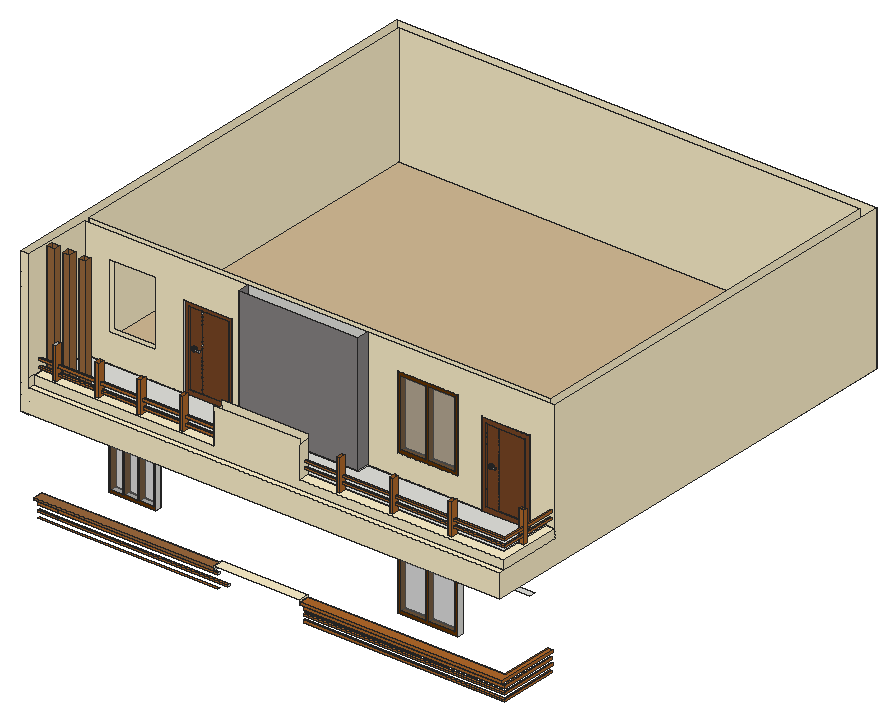
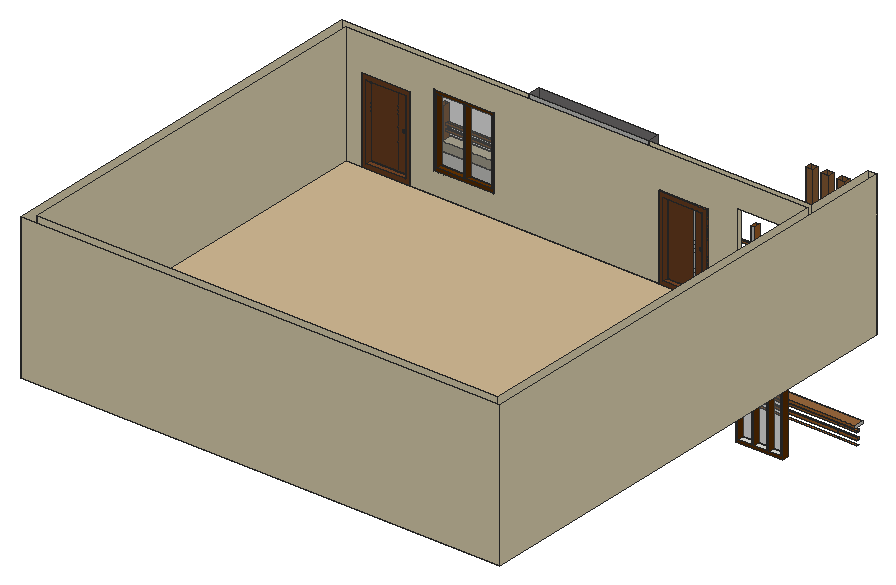
# SketchUp Ruby script. Lengths in inches.
U = 1.inch
M = Sketchup.active_model
def pt(a) = Geom::Point3d.new(a.map { |v| v * U })
def face(e, loops, mat)
  f = e.add_face(loops[0].map { |a| pt(a) })
  loops[1..].each { |l| e.add_face(l.map { |a| pt(a) }).erase! }
  f.material = f.back_material = mat if mat
  f
end
# faces: each face lists its corners as indices into pts; further lists are holes
def faces(e, pts, list, mat = nil) = list.each { |f| face(e, (f[0].is_a?(Array) ? f : [f]).map { |l| l.map { |i| pts[i] } }, mat) }
# xy, xz, yz: faces in a plane at the given z, y or x. An outline is a flat list of corners, or four numbers for a rectangle; further outlines are holes
def ring(l) = l.size == 4 ? [[l[0], l[1]], [l[2], l[1]], [l[2], l[3]], [l[0], l[3]]] : l.each_slice(2).to_a
def flat(e, list, mat, &to3) = list.each { |f| face(e, (f[0].is_a?(Array) ? f : [f]).map { |l| ring(l).map { |u, v| to3.(u, v) } }, mat) }
def xy(e, z, list, mat = nil) = flat(e, list, mat) { |x, y| [x, y, z] }
def xz(e, y, list, mat = nil) = flat(e, list, mat) { |x, z| [x, y, z] }
def yz(e, x, list, mat = nil) = flat(e, list, mat) { |y, z| [x, y, z] }
def lines(e, pts, list) = list.each { |a, b| e.add_line(pt(pts[a]), pt(pts[b])) }
# prism: a flat outline (further loops are holes) pulled along v
def prism(e, loops, v, mat = nil)
  f = face(e, loops, mat); d = Geom::Vector3d.new(v.map { |x| x * U })
  f.pushpull(f.normal.samedirection?(d) ? d.length : -d.length)
end
def box(e, o, s, mat = nil) = prism(e, [[o, [o[0] + s[0], o[1], o[2]], [o[0] + s[0], o[1] + s[1], o[2]], [o[0], o[1] + s[1], o[2]]]], [0, 0, s[2]], mat)
def at(x, y, z, deg = 0) = Geom::Transformation.translation(pt([x, y, z])) * Geom::Transformation.rotation(ORIGIN, Z_AXIS, deg.degrees)
def axes(o, x, y, z) = Geom::Transformation.new([*x, 0, *y, 0, *z, 0, *pt(o).to_a, 1])
def part(name) = M.definitions.add(name)
# library, detail: a bought-in or finely detailed component or shape, given as its bounding box
def library(name, o, s) = part(name).tap { |d| box(d.entities, o, s) }
def detail(e, o, s) = box(e.add_group.entities, o, s)
def put(e, d, t, mat = nil) = e.add_instance(d, t).tap { |i| i.material = mat if mat }
def group(e, t, mat = nil) = e.add_group.tap { |g| g.transformation = t; g.material = mat if mat }.entities
root = M.entities
M.materials.add("[Aluminum]").color = [179, 179, 179]
M.materials.add("[Brick Tumbled]").color = [135, 132, 132]
M.materials.add("[Color C08]").color = [102, 51, 0]
M.materials.add("[Color D01]").color = [255, 242, 204]
M.materials.add("[Formica Beige]").color = [211, 187, 149]
M.materials.add("[Translucent Glass Gray]").color = [128, 128, 128]
M.materials["[Translucent Glass Gray]"].alpha = 0.5
M.materials.add("[Wood Bamboo]").color = [177, 105, 43]
M.materials.add("[Wood Floor]").color = [155, 105, 61]
M.materials.add("[Wood Veneer 01]").color = [120, 70, 37]
c1 = part("Group\#4")
xy(c1.entities,0,[[0,0,52.875,9]],"[Color C08]")
xy(c1.entities,2.31,[[2.31,0,24.96,9],[26.98,0,50.56,9]],"[Color C08]")
xy(c1.entities,50.56,[[2.31,0,24.96,9],[26.98,0,50.56,9]],"[Color C08]")
xy(c1.entities,52.875,[[0,0,52.875,9]],"[Color C08]")
xz(c1.entities,0,[[[0,0,52.875,52.875],[26.98,2.31,50.56,50.56],[2.31,2.31,24.96,50.56]]],"[Color C08]")
xz(c1.entities,0,[[2.31,2.31,24.96,50.56],[26.98,2.31,50.56,50.56]],"[Translucent Glass Gray]")
xz(c1.entities,9,[[[0,0,52.875,52.875],[26.98,2.31,50.56,50.56],[2.31,2.31,24.96,50.56]]],"[Color C08]")
yz(c1.entities,0,[[0,0,9,52.875]],"[Color C08]")
yz(c1.entities,2.31,[[0,2.31,9,50.56]],"[Color C08]")
yz(c1.entities,24.96,[[0,2.31,9,50.56]],"[Color C08]")
yz(c1.entities,26.98,[[0,2.31,9,50.56]],"[Color C08]")
yz(c1.entities,50.56,[[0,2.31,9,50.56]],"[Color C08]")
yz(c1.entities,52.875,[[0,0,9,52.875]],"[Color C08]")
xy(root,309.67,[[322.9,204.4,382.78,210.4]])
xy(root,310.18,[[274.98,145.89,274.98,148.02,475.1875,148.02,475.1875,204.4,477.01,204.4,477.01,145.89]],"[Wood Bamboo]")
xy(root,310.55,[[9,146.02,28.82,148.14],[28.82,146.02,189.63,148.14]],"[Wood Bamboo]")
xy(root,312.3,[[274.98,145.89,477.01,145.89,477.01,204.4,475.1875,204.4,475.1875,148.02,274.98,148.02]],"[Wood Bamboo]")
xy(root,315.61,[[9,146.02,28.82,148.14]])
xy(root,315.61,[[28.82,146.02,199.2,148.14]],"[Wood Bamboo]")
xy(root,316.36,[[274.98,145.89,274.98,148.02,475.1875,148.02,475.1875,205.64,477.01,205.64,477.01,145.89]],"[Wood Bamboo]")
xy(root,316.68,[[33.82,204.4,80.13,210.4]])
xy(root,317.73,[[9,146.02,28.82,148.14],[28.82,146.02,199.2,148.14]],"[Wood Bamboo]")
xy(root,318.49,[[274.98,145.89,477.01,145.89,477.01,205.64,475.1875,205.64,475.1875,148.02,274.98,148.02]],"[Wood Bamboo]")
xy(root,321.93,[[274.98,145.89,274.98,148.02,475.1875,148.02,475.1875,204.36,477.01,204.36,477.01,145.89]],"[Wood Bamboo]")
xy(root,322.48,[[9,146.02,28.82,148.14]])
xy(root,322.48,[[28.82,146.02,189.2,148.14]],"[Wood Bamboo]")
xy(root,324.43,[[274.98,145.89,477.01,145.89,477.01,204.36,475.1875,204.36,475.1875,148.02,274.98,148.02]],"[Wood Bamboo]")
xy(root,324.61,[[9,146.02,28.82,148.14],[28.82,146.02,189.2,148.14]],"[Wood Bamboo]")
xy(root,327.9375,[[309.7,143.88,313.07,150.13]])
xy(root,328.12,[[[8.16,141.71,188.91,151.78],[68.13,143.88,71.51,150.13],[110.26,143.88,113.63,150.13]],[[274.98,141.71,274.98,151.78,472.375,151.78,472.375,205.65,477.34,205.65,477.34,141.71],[421.51,143.88,424.88,150.13]]],"[Wood Bamboo]")
xy(root,328.125,[[472.3125,168.86,477.25,172.24]])
xy(root,328.375,[[152.95,143.88,156.32,150.13]])
xy(root,328.5,[[362.95,143.88,366.32,150.13]])
xy(root,328.9375,[[25.45,143.88,28.82,150.13]])
xy(root,330.66,[[274.98,141.71,477.34,141.71,477.34,205.65,472.375,205.65,472.375,151.78,274.98,151.78]],"[Wood Bamboo]")
xy(root,330.66,[[8.16,141.71,188.91,151.78]],"[Wood Floor]")
xy(root,332.875,[[188.91,140.9,274.98,151.78]],"[Color D01]")
xy(root,371.875,[[108.75,204.4,156.75,210.4],[407.0625,204.4,455.0625,210.4]])
xy(root,382.5,[[33.82,204.4,80.13,210.4]])
xy(root,382.8,[[322.9,204.4,382.78,210.4]])
xy(root,407.875,[[0,135.4,480,606.75]])
xy(root,407.875,[[172.75,192.4,292.75,204.4]],"[Brick Tumbled]")
xy(root,407.875,[[[0,135.4,9,135.4,9,204.4,480,204.4,480,606.75,0,606.75],[9,210.4,471,597.75]]],"[Color D01]")
xy(root,407.875,[[11.75,154.17,19.6875,160.61],[27.8125,154.17,35,160.61],[43.5625,154.17,50.1875,160.61]],"[Wood Floor]")
xy(root,420.875,[[9,151.78,9,204.4,108.75,204.4,108.75,210.4,156.75,210.4,156.75,204.4,172.75,204.4,172.75,192.4,292.75,192.4,292.75,204.4,407.0625,204.4,407.0625,210.4,455.0625,210.4,455.0625,204.4,471,204.4,471,151.78]])
xy(root,431.8125,[[9,140.9,9,151.78,471,151.78,471,204.4,480,204.4,480,140.9],[[9,151.78,471,151.78,471,204.4,455.0625,204.4,455.0625,210.4,407.0625,210.4,407.0625,204.4,292.75,204.4,292.75,192.4,172.75,192.4,172.75,204.4,156.75,204.4,156.75,210.4,108.75,210.4,108.75,204.4,9,204.4],[11.75,154.17,19.6875,160.61],[27.8125,154.17,35,160.61],[43.5625,154.17,50.1875,160.61]],[172.75,192.4,292.75,204.4],[156.75,204.4,407.0625,210.4]])
xy(root,431.8125,[[9,135.4,480,140.9]],"[Color D01]")
xy(root,431.8125,[[9,210.4,471,597.75]],"[Formica Beige]")
xy(root,440.8125,[[[9,140.9,188.91,151.78],[25.45,143.88,28.82,150.13],[68.13,143.88,71.51,150.13],[110.26,143.88,113.63,150.13],[152.95,143.88,156.32,150.13]],[[274.98,140.9,480,140.9,480,204.4,471,204.4,471,151.78,274.98,151.78],[309.7,143.88,313.07,150.13],[421.51,143.88,424.88,150.13],[362.95,143.88,366.32,150.13],[472.3125,168.86,477.25,172.24]]],"[Color D01]")
xy(root,445.02,[[9,146.22,28.82,148.34]])
xy(root,445.02,[[28.82,146.22,188.91,148.34]],"[Wood Bamboo]")
xy(root,447.15,[[9,146.22,28.82,148.34],[28.82,146.22,188.91,148.34]],"[Wood Bamboo]")
xy(root,447.99,[[274.98,145.89,274.98,148.02,475.1875,148.02,475.1875,207.71,477.01,207.71,477.01,145.89]],"[Wood Bamboo]")
xy(root,450.11,[[274.98,145.89,477.01,145.89,477.01,207.71,475.1875,207.71,475.1875,148.02,274.98,148.02]],"[Wood Bamboo]")
xy(root,452.36,[[9,146.02,28.82,148.14]])
xy(root,452.36,[[28.82,146.02,189.63,148.14]],"[Wood Bamboo]")
xy(root,453.61,[[322.9,204.4,382.78,210.4]])
xy(root,454.11,[[274.98,145.89,274.98,148.02,475.1875,148.02,475.1875,204.4,477.01,204.4,477.01,145.89]],"[Wood Bamboo]")
xy(root,454.48,[[9,146.02,28.82,148.14],[28.82,146.02,189.63,148.14]],"[Wood Bamboo]")
xz(root,135.4,[[0,407.875,480,407.875,480,431.8125,9,431.8125,9,551.8125,0,551.8125]],"[Color D01]")
xz(root,140.9,[[9,431.8125,480,431.8125,480,440.8125,274.98,440.8125,274.98,476.8125,188.91,476.8125,188.91,440.8125,9,440.8125]],"[Color D01]")
xz(root,141.71,[[274.98,328.12,477.34,330.66]],"[Wood Bamboo]")
xz(root,141.71,[[8.16,328.12,188.91,330.66]],"[Wood Floor]")
xz(root,143.88,[[25.45,440.8125,28.82,472.875],[68.13,440.8125,71.51,472.05],[110.26,440.8125,113.63,472.05],[152.95,440.8125,156.32,472.3125],[309.7,440.8125,313.07,471.875],
  [362.95,440.8125,366.32,472.4375],[421.51,440.8125,424.88,472.05]],"[Wood Bamboo]")
xz(root,145.89,[[274.98,310.18,477.01,312.3],[274.98,316.36,477.01,318.49],[274.98,321.93,477.01,324.43],[274.98,447.99,477.01,450.11],[274.98,454.11,477.01,456.24]],"[Wood Bamboo]")
xz(root,146.02,[[9,315.61,28.82,317.73],[28.82,315.61,199.2,317.73],[9,322.48,28.82,324.61],[28.82,322.48,189.2,324.61],[9,452.36,28.82,454.48],
  [28.82,452.36,189.63,454.48]],"[Wood Bamboo]")
xz(root,146.22,[[9,445.02,28.82,447.15],[28.82,445.02,188.91,447.15]],"[Wood Bamboo]")
xz(root,148.02,[[274.98,310.18,475.1875,312.3],[274.98,316.36,475.1875,318.49],[274.98,321.93,475.1875,324.43],[274.98,447.99,475.1875,450.11],[274.98,454.11,475.1875,456.24]],"[Wood Bamboo]")
xz(root,148.14,[[9,315.61,28.82,317.73],[28.82,315.61,199.2,317.73],[9,322.48,28.82,324.61],[28.82,322.48,189.2,324.61],[9,452.36,28.82,454.48],
  [28.82,452.36,189.63,454.48]],"[Wood Bamboo]")
xz(root,148.34,[[9,445.02,28.82,447.15],[28.82,445.02,188.91,447.15]],"[Wood Bamboo]")
xz(root,150.13,[[110.26,440.8125,113.63,472.05],[152.95,440.8125,156.32,472.3125]])
xz(root,150.13,[[25.45,440.8125,28.82,472.875],[68.13,440.8125,71.51,472.05],[309.7,440.8125,313.07,471.875],[362.95,440.8125,366.32,472.4375],[421.51,440.8125,424.88,472.05]],"[Wood Bamboo]")
xz(root,151.78,[[9,420.875,471,431.8125]])
xz(root,151.78,[[9,431.8125,9,440.8125,188.91,440.8125,188.91,476.8125,274.98,476.8125,274.98,440.8125,471,440.8125,471,431.8125]],"[Color D01]")
xz(root,151.78,[[8.16,328.12,188.91,330.66],[274.98,328.12,472.375,330.66]],"[Wood Bamboo]")
xz(root,154.17,[[11.75,431.8125,19.6875,551.8125],[27.8125,431.8125,35,551.8125],[43.5625,431.8125,50.1875,551.8125]],"[Wood Floor]")
xz(root,160.61,[[11.75,431.8125,19.6875,551.8125],[27.8125,431.8125,35,551.8125],[43.5625,431.8125,50.1875,551.8125]],"[Wood Floor]")
xz(root,168.86,[[472.3125,440.8125,477.25,472.0625]],"[Wood Bamboo]")
xz(root,172.24,[[472.3125,440.8125,477.25,472.0625]],"[Wood Bamboo]")
xz(root,192.4,[[172.75,420.875,292.75,431.8125]])
xz(root,192.4,[[172.75,431.8125,292.75,551.8125]],"[Brick Tumbled]")
xz(root,204.36,[[475.1875,321.93,477.01,324.43]])
xz(root,204.4,[[9,420.875,108.75,431.8125],[156.75,420.875,172.75,431.8125],[292.75,420.875,407.0625,431.8125],[455.0625,420.875,471,431.8125],[172.75,431.8125,292.75,551.8125],
  [471,431.8125,480,440.8125]])
xz(root,204.4,[[[9,431.8125,108.75,431.8125,108.75,515.8125,156.75,515.8125,156.75,431.8125,172.75,431.8125,172.75,551.8125,9,551.8125],[33.82,460.62,80.13,526.43]],[[292.75,431.8125,407.0625,431.8125,407.0625,515.8125,455.0625,515.8125,455.0625,431.8125,471,431.8125,471,440.8125,480,440.8125,480,551.8125,292.75,551.8125],[322.9,453.61,382.78,526.73],[475.1875,454.11,477.01,456.24]]],"[Color D01]")
xz(root,205.64,[[475.1875,316.36,477.01,318.49]])
xz(root,205.65,[[472.375,328.12,477.34,330.66]])
xz(root,207.71,[[475.1875,447.99,477.01,450.11]])
xz(root,210.4,[[108.75,420.875,156.75,431.8125],[407.0625,420.875,455.0625,431.8125]])
xz(root,210.4,[[[9,431.8125,9,551.8125,471,551.8125,471,431.8125,455.0625,431.8125,455.0625,515.8125,407.0625,515.8125,407.0625,431.8125,156.75,431.8125,156.75,515.8125,108.75,515.8125,108.75,431.8125],[322.9,453.61,382.78,526.73],[33.82,460.62,80.13,526.43]]],"[Color D01]")
xz(root,597.75,[[9,431.8125,471,551.8125]],"[Color D01]")
xz(root,606.75,[[0,407.875,480,551.8125]],"[Color D01]")
yz(root,0,[[135.4,407.875,606.75,551.8125]],"[Color D01]")
yz(root,8.16,[[141.71,328.12,151.78,330.66]])
yz(root,9,[[151.78,420.875,204.4,431.8125],[140.9,431.8125,151.78,440.8125]])
yz(root,9,[[135.4,431.8125,140.9,440.8125],[[151.78,431.8125,204.4,431.8125,204.4,551.8125,135.4,551.8125,135.4,440.8125,151.78,440.8125],[146.02,466.42,148.14,468.55],[146.02,459.55,148.14,461.67],[146.02,452.36,148.14,454.48],[146.22,445.02,148.34,447.15]],[210.4,431.8125,597.75,551.8125]],"[Color D01]")
yz(root,11.75,[[154.17,431.8125,160.61,551.8125]],"[Wood Floor]")
yz(root,19.6875,[[154.17,431.8125,160.61,551.8125]],"[Wood Floor]")
yz(root,25.45,[[143.88,440.8125,150.13,472.875]])
yz(root,27.8125,[[154.17,431.8125,160.61,551.8125]],"[Wood Floor]")
yz(root,28.82,[[146.02,315.61,148.14,317.73],[146.02,322.48,148.14,324.61],[146.22,445.02,148.34,447.15],[146.02,452.36,148.14,454.48]])
yz(root,28.82,[[[143.88,440.8125,150.13,472.875],[146.02,466.42,148.14,468.55],[146.02,459.55,148.14,461.67],[146.02,452.36,148.14,454.48],[146.22,445.02,148.34,447.15]]],"[Wood Bamboo]")
yz(root,33.82,[[204.4,316.68,210.4,382.5]])
yz(root,35,[[154.17,431.8125,160.61,551.8125]],"[Wood Floor]")
yz(root,43.5625,[[154.17,431.8125,160.61,551.8125]],"[Wood Floor]")
yz(root,50.1875,[[154.17,431.8125,160.61,551.8125]],"[Wood Floor]")
yz(root,68.13,[[143.88,440.8125,150.13,472.05]],"[Wood Bamboo]")
yz(root,71.51,[[143.88,440.8125,150.13,472.05]],"[Wood Bamboo]")
yz(root,80.13,[[204.4,316.68,210.4,382.5]])
yz(root,108.75,[[204.4,420.875,210.4,431.8125],[204.4,431.8125,210.4,515.8125]])
yz(root,110.26,[[143.88,440.8125,150.13,472.05]],"[Wood Bamboo]")
yz(root,113.63,[[143.88,440.8125,150.13,472.05]],"[Wood Bamboo]")
yz(root,152.95,[[143.88,440.8125,150.13,472.3125]],"[Wood Bamboo]")
yz(root,156.32,[[143.88,440.8125,150.13,472.3125]],"[Wood Bamboo]")
yz(root,156.75,[[204.4,420.875,210.4,431.8125],[204.4,431.8125,210.4,515.8125]])
yz(root,172.75,[[192.4,420.875,204.4,431.8125]])
yz(root,172.75,[[192.4,431.8125,204.4,551.8125]],"[Brick Tumbled]")
yz(root,188.91,[[141.71,328.12,151.78,330.66]])
yz(root,188.91,[[140.9,328.12,141.71,330.66],[140.9,330.66,151.78,332.875],[[140.9,440.8125,151.78,472.05],[146.22,445.02,148.34,447.15]]],"[Color D01]")
yz(root,189.2,[[146.02,322.48,148.14,324.61]])
yz(root,189.63,[[146.02,452.36,148.14,454.48]])
yz(root,199.2,[[146.02,315.61,148.14,317.73]])
yz(root,274.98,[[141.71,328.12,151.78,330.66]])
yz(root,274.98,[[140.9,328.12,141.71,330.66],[140.9,330.66,151.78,332.875],[[140.9,440.8125,151.78,472.05],[145.89,465.86,148.02,468.36],[145.89,460.3,148.02,462.43],[145.89,454.11,148.02,456.24],[145.89,447.99,148.02,450.11]]],"[Color D01]")
yz(root,292.75,[[192.4,420.875,204.4,431.8125]])
yz(root,292.75,[[192.4,431.8125,204.4,551.8125]],"[Brick Tumbled]")
yz(root,309.7,[[143.88,440.8125,150.13,471.875]],"[Wood Bamboo]")
yz(root,313.07,[[143.88,440.8125,150.13,471.875]],"[Wood Bamboo]")
yz(root,322.9,[[204.4,309.67,210.4,382.8],[204.4,453.61,210.4,526.73]])
yz(root,362.95,[[143.88,440.8125,150.13,472.4375]],"[Wood Bamboo]")
yz(root,366.32,[[143.88,440.8125,150.13,472.4375]],"[Wood Bamboo]")
yz(root,382.78,[[204.4,309.67,210.4,382.8],[204.4,453.61,210.4,526.73]])
yz(root,407.0625,[[204.4,420.875,210.4,431.8125],[204.4,431.8125,210.4,515.8125]])
yz(root,421.51,[[143.88,440.8125,150.13,472.05]],"[Wood Bamboo]")
yz(root,424.88,[[143.88,440.8125,150.13,472.05]],"[Wood Bamboo]")
yz(root,455.0625,[[204.4,420.875,210.4,431.8125],[204.4,431.8125,210.4,515.8125]])
yz(root,471,[[151.78,420.875,204.4,431.8125]])
yz(root,471,[[151.78,431.8125,204.4,440.8125],[210.4,431.8125,597.75,551.8125]],"[Color D01]")
yz(root,472.3125,[[168.86,440.8125,172.24,472.0625]],"[Wood Bamboo]")
yz(root,472.375,[[151.78,328.12,205.65,330.66]],"[Wood Bamboo]")
yz(root,475.1875,[[148.02,310.18,204.4,312.3],[148.02,316.36,205.64,318.49],[148.02,321.93,204.36,324.43],[148.02,447.99,207.71,450.11],[148.02,454.11,204.4,456.24]],"[Wood Bamboo]")
yz(root,477.01,[[145.89,310.18,204.4,312.3],[145.89,316.36,205.64,318.49],[145.89,321.93,204.36,324.43],[145.89,447.99,207.71,450.11],[145.89,454.11,204.4,456.24]],"[Wood Bamboo]")
yz(root,477.25,[[168.86,440.8125,172.24,472.0625]],"[Wood Bamboo]")
yz(root,477.34,[[141.71,328.12,205.65,330.66]],"[Wood Bamboo]")
yz(root,480,[[135.4,407.875,606.75,407.875,606.75,551.8125,204.4,551.8125,204.4,431.8125,135.4,431.8125],[140.9,431.8125,204.4,440.8125]],"[Color D01]")
p = [[9,597.75,419.8125],[9,597.75,431.8125],[9,204.4,419.8125],[9,204.4,420.875],[471,204.4,419.8125],[471,204.4,420.875],
  [9,144.4,419.8125],[9,135.4,419.8125],[9,210.4,419.8125],[9,210.4,431.8125],[9,144.4,431.8125],[471,597.75,419.8125],
  [471,597.75,431.8125],[471,210.4,419.8125],[471,210.4,431.8125]]
lines(root,p,[[0,1],[2,3],[4,5],[6,7],[8,9],[6,10],[11,12],[13,14]])
put(root,c1,axes([322.9,204.4,309.67],[1.13239,0,0],[0,0.62,0],[0,0,1.38298]))
g1 = group(root,at(33.75,204.4,316.68))
xy(g1,0,[[0,0,46.38,6.12]],"[Color C08]")
xy(g1,2.88,[[2.03,0,13.84,6.12],[15.61,0,28.92,6.12],[30.6875,0,44.35,6.12]])
xy(g1,62.93,[[2.03,0,13.84,6.12],[15.61,0,28.92,6.12],[30.6875,0,44.35,6.12]],"[Color C08]")
xy(g1,65.8125,[[0,0,46.38,6.12]],"[Color C08]")
xz(g1,0,[[[0,0,46.38,65.8125],[30.6875,2.88,44.35,62.93],[15.61,2.88,28.92,62.93],[2.03,2.88,13.84,62.93]]],"[Color C08]")
xz(g1,0,[[2.03,2.88,13.84,62.93],[15.61,2.88,28.92,62.93],[30.6875,2.88,44.35,62.93]],"[Translucent Glass Gray]")
xz(g1,6.12,[[[0,0,46.38,65.8125],[30.6875,2.88,44.35,62.93],[15.61,2.88,28.92,62.93],[2.03,2.88,13.84,62.93]]],"[Color C08]")
yz(g1,0,[[0,0,6.12,65.8125]],"[Color C08]")
yz(g1,2.03,[[0,2.88,6.12,62.93]],"[Color C08]")
yz(g1,13.84,[[0,2.88,6.12,62.93]],"[Color C08]")
yz(g1,15.61,[[0,2.88,6.12,62.93]],"[Color C08]")
yz(g1,28.92,[[0,2.88,6.12,62.93]],"[Color C08]")
yz(g1,30.6875,[[0,2.88,6.12,62.93]],"[Color C08]")
yz(g1,44.35,[[0,2.88,6.12,62.93]],"[Color C08]")
yz(g1,46.38,[[0,0,6.12,65.8125]],"[Color C08]")
g2 = group(root,at(407.0625,202.84,431.8125))
xy(g2,0,[[0,1.02,48,1.91],[0,1.91,48,7.76]],"[Wood Veneer 01]")
xy(g2,4.26,[[4.26,1.02,43.74,1.91],[4.26,1.91,43.74,7.76]],"[Wood Veneer 01]")
xy(g2,41.66,[[8.83,0,8.83,0.93,9.58,0.93,9.58,0.47,15.08,0.47,15.08,0]],"[Aluminum]")
xy(g2,43.35,[[8.83,0,15.08,0,15.08,0.47,9.58,0.47,9.58,0.93,8.83,0.93]],"[Aluminum]")
xy(g2,79.74,[[4.26,1.02,16.16,1.91],[16.16,1.02,16.99,1.91],[16.99,1.02,43.74,1.91],[4.26,1.91,43.74,7.76]],"[Wood Veneer 01]")
xy(g2,84,[[0,1.02,48,1.91],[0,1.91,48,7.76]],"[Wood Veneer 01]")
xz(g2,0,[[8.83,41.66,15.08,43.35]],"[Aluminum]")
xz(g2,0.47,[[9.58,41.66,15.08,43.35]],"[Aluminum]")
xz(g2,0.93,[[[9.24,40.44,9.77,40.51,10.27,40.72,10.7,41.05,11.03,41.47,11.23,41.97,11.3,42.5,11.23,43.04,11.03,43.54,10.7,43.96,10.27,44.29,9.77,44.5,9.24,44.57,8.71,44.5,8.21,44.29,7.78,43.96,7.45,43.54,7.25,43.04,7.18,42.5,7.25,41.97,7.45,41.47,7.78,41.05,8.21,40.72,8.71,40.51],[8.83,41.66,9.58,43.35]]],"[Aluminum]")
xz(g2,1.02,[[[0,0,48,84],[4.26,4.26,43.74,79.74]]],"[Wood Veneer 01]")
xz(g2,1.91,[[[0,0,48,84],[4.26,4.26,43.74,79.74]],[16.16,4.26,16.99,79.74]])
xz(g2,1.91,[[[4.26,4.26,16.16,79.74],[9.24,40.44,8.71,40.51,8.21,40.72,7.78,41.05,7.45,41.47,7.25,41.97,7.18,42.5,7.25,43.04,7.45,43.54,7.78,43.96,8.21,44.29,8.71,44.5,9.24,44.57,9.77,44.5,10.27,44.29,10.7,43.96,11.03,43.54,11.23,43.04,11.3,42.5,11.23,41.97,11.03,41.47,10.7,41.05,10.27,40.72,9.77,40.51]],[16.99,4.26,43.74,79.74]],"[Wood Veneer 01]")
xz(g2,7.76,[[[0,0,48,84],[4.26,4.26,43.74,79.74]]],"[Wood Veneer 01]")
yz(g2,0,[[1.02,0,1.91,84],[1.91,0,7.76,84]],"[Wood Veneer 01]")
yz(g2,4.26,[[1.02,4.26,1.91,79.74],[1.91,4.26,7.76,79.74]],"[Wood Veneer 01]")
yz(g2,8.83,[[0,41.66,0.93,43.35]],"[Aluminum]")
yz(g2,9.58,[[0.47,41.66,0.93,43.35]],"[Aluminum]")
yz(g2,15.08,[[0,41.66,0.47,43.35]],"[Aluminum]")
yz(g2,43.74,[[1.02,4.26,1.91,79.74],[1.91,4.26,7.76,79.74]],"[Wood Veneer 01]")
yz(g2,48,[[1.02,0,1.91,84],[1.91,0,7.76,84]],"[Wood Veneer 01]")
p = [[8.71,1.91,40.51],[9.24,1.91,40.44],[9.24,0.93,40.44],[8.71,0.93,40.51],[9.77,1.91,40.51],[9.77,0.93,40.51],
  [8.21,1.91,40.72],[8.21,0.93,40.72],[10.27,1.91,40.72],[10.27,0.93,40.72],[7.78,1.91,41.05],[7.78,0.93,41.05],
  [10.7,1.91,41.05],[10.7,0.93,41.05],[7.45,1.91,41.47],[7.45,0.93,41.47],[11.03,1.91,41.47],[11.03,0.93,41.47],
  [7.25,1.91,41.97],[7.25,0.93,41.97],[11.23,1.91,41.97],[11.23,0.93,41.97],[7.18,1.91,42.5],[7.18,0.93,42.5],
  [11.3,1.91,42.5],[11.3,0.93,42.5],[7.25,1.91,43.04],[7.25,0.93,43.04],[11.23,1.91,43.04],[11.23,0.93,43.04],
  [7.45,1.91,43.54],[7.45,0.93,43.54],[11.03,1.91,43.54],[11.03,0.93,43.54],[7.78,1.91,43.96],[7.78,0.93,43.96],
  [10.7,1.91,43.96],[10.7,0.93,43.96],[8.21,1.91,44.29],[8.21,0.93,44.29],[10.27,1.91,44.29],[10.27,0.93,44.29],
  [8.71,1.91,44.5],[8.71,0.93,44.5],[9.77,1.91,44.5],[9.77,0.93,44.5],[9.24,1.91,44.57],[9.24,0.93,44.57]]
faces(g2,p,[[0,1,2,3],[1,4,5,2],[6,0,3,7],[4,8,9,5],[10,6,7,11],[8,12,13,9],[14,10,11,15],[12,16,17,13],
  [18,14,15,19],[16,20,21,17],[22,18,19,23],[20,24,25,21],[26,22,23,27],[24,28,29,25],[30,26,27,31],[28,32,33,29],
  [34,30,31,35],[32,36,37,33],[38,34,35,39],[36,40,41,37],[42,38,39,43],[40,44,45,41],[46,42,43,47],[44,46,47,45]],"[Aluminum]")
g3 = group(root,at(108.75,204.4,431.8125))
xy(g3,0,[[0,1.02,48,1.91],[0,1.91,48,7.76]],"[Wood Veneer 01]")
xy(g3,4.26,[[4.26,1.02,43.74,1.91],[4.26,1.91,43.74,7.76]],"[Wood Veneer 01]")
xy(g3,41.66,[[8.83,0,8.83,0.93,9.58,0.93,9.58,0.47,15.08,0.47,15.08,0]],"[Aluminum]")
xy(g3,43.35,[[8.83,0,15.08,0,15.08,0.47,9.58,0.47,9.58,0.93,8.83,0.93]],"[Aluminum]")
xy(g3,79.74,[[4.26,1.02,16.16,1.91],[16.16,1.02,16.99,1.91],[16.99,1.02,43.74,1.91],[4.26,1.91,43.74,7.76]],"[Wood Veneer 01]")
xy(g3,84,[[0,1.02,48,1.91],[0,1.91,48,7.76]],"[Wood Veneer 01]")
xz(g3,0,[[8.83,41.66,15.08,43.35]],"[Aluminum]")
xz(g3,0.47,[[9.58,41.66,15.08,43.35]],"[Aluminum]")
xz(g3,0.93,[[[9.24,40.44,9.77,40.51,10.27,40.72,10.7,41.05,11.03,41.47,11.23,41.97,11.3,42.5,11.23,43.04,11.03,43.54,10.7,43.96,10.27,44.29,9.77,44.5,9.24,44.57,8.71,44.5,8.21,44.29,7.78,43.96,7.45,43.54,7.25,43.04,7.18,42.5,7.25,41.97,7.45,41.47,7.78,41.05,8.21,40.72,8.71,40.51],[8.83,41.66,9.58,43.35]]],"[Aluminum]")
xz(g3,1.02,[[[0,0,48,84],[4.26,4.26,43.74,79.74]]],"[Wood Veneer 01]")
xz(g3,1.91,[[[0,0,48,84],[4.26,4.26,43.74,79.74]],[16.16,4.26,16.99,79.74]])
xz(g3,1.91,[[[4.26,4.26,16.16,79.74],[9.24,40.44,8.71,40.51,8.21,40.72,7.78,41.05,7.45,41.47,7.25,41.97,7.18,42.5,7.25,43.04,7.45,43.54,7.78,43.96,8.21,44.29,8.71,44.5,9.24,44.57,9.77,44.5,10.27,44.29,10.7,43.96,11.03,43.54,11.23,43.04,11.3,42.5,11.23,41.97,11.03,41.47,10.7,41.05,10.27,40.72,9.77,40.51]],[16.99,4.26,43.74,79.74]],"[Wood Veneer 01]")
xz(g3,7.76,[[[0,0,48,84],[4.26,4.26,43.74,79.74]]],"[Wood Veneer 01]")
yz(g3,0,[[1.02,0,1.91,84],[1.91,0,7.76,84]],"[Wood Veneer 01]")
yz(g3,4.26,[[1.02,4.26,1.91,79.74],[1.91,4.26,7.76,79.74]],"[Wood Veneer 01]")
yz(g3,8.83,[[0,41.66,0.93,43.35]],"[Aluminum]")
yz(g3,9.58,[[0.47,41.66,0.93,43.35]],"[Aluminum]")
yz(g3,15.08,[[0,41.66,0.47,43.35]],"[Aluminum]")
yz(g3,43.74,[[1.02,4.26,1.91,79.74],[1.91,4.26,7.76,79.74]],"[Wood Veneer 01]")
yz(g3,48,[[1.02,0,1.91,84],[1.91,0,7.76,84]],"[Wood Veneer 01]")
p = [[8.71,1.91,40.51],[9.24,1.91,40.44],[9.24,0.93,40.44],[8.71,0.93,40.51],[9.77,1.91,40.51],[9.77,0.93,40.51],
  [8.21,1.91,40.72],[8.21,0.93,40.72],[10.27,1.91,40.72],[10.27,0.93,40.72],[7.78,1.91,41.05],[7.78,0.93,41.05],
  [10.7,1.91,41.05],[10.7,0.93,41.05],[7.45,1.91,41.47],[7.45,0.93,41.47],[11.03,1.91,41.47],[11.03,0.93,41.47],
  [7.25,1.91,41.97],[7.25,0.93,41.97],[11.23,1.91,41.97],[11.23,0.93,41.97],[7.18,1.91,42.5],[7.18,0.93,42.5],
  [11.3,1.91,42.5],[11.3,0.93,42.5],[7.25,1.91,43.04],[7.25,0.93,43.04],[11.23,1.91,43.04],[11.23,0.93,43.04],
  [7.45,1.91,43.54],[7.45,0.93,43.54],[11.03,1.91,43.54],[11.03,0.93,43.54],[7.78,1.91,43.96],[7.78,0.93,43.96],
  [10.7,1.91,43.96],[10.7,0.93,43.96],[8.21,1.91,44.29],[8.21,0.93,44.29],[10.27,1.91,44.29],[10.27,0.93,44.29],
  [8.71,1.91,44.5],[8.71,0.93,44.5],[9.77,1.91,44.5],[9.77,0.93,44.5],[9.24,1.91,44.57],[9.24,0.93,44.57]]
faces(g3,p,[[0,1,2,3],[1,4,5,2],[6,0,3,7],[4,8,9,5],[10,6,7,11],[8,12,13,9],[14,10,11,15],[12,16,17,13],
  [18,14,15,19],[16,20,21,17],[22,18,19,23],[20,24,25,21],[26,22,23,27],[24,28,29,25],[30,26,27,31],[28,32,33,29],
  [34,30,31,35],[32,36,37,33],[38,34,35,39],[36,40,41,37],[42,38,39,43],[40,44,45,41],[46,42,43,47],[44,46,47,45]],"[Aluminum]")
g4 = group(root,at(322.9,204.4,453.61))
xy(g4,0,[[0,0,59.875,5.58]],"[Color C08]")
xy(g4,3.2,[[2.62,0,28.27,5.58],[30.56,0,57.25,5.58]],"[Color C08]")
xy(g4,69.92,[[2.62,0,28.27,5.58],[30.56,0,57.25,5.58]],"[Color C08]")
xy(g4,73.125,[[0,0,59.875,5.58]],"[Color C08]")
xz(g4,0,[[[0,0,59.875,73.125],[30.56,3.2,57.25,69.92],[2.62,3.2,28.27,69.92]]],"[Color C08]")
xz(g4,0,[[2.62,3.2,28.27,69.92],[30.56,3.2,57.25,69.92]],"[Translucent Glass Gray]")
xz(g4,5.58,[[[0,0,59.875,73.125],[30.56,3.2,57.25,69.92],[2.62,3.2,28.27,69.92]]],"[Color C08]")
yz(g4,0,[[0,0,5.58,73.125]],"[Color C08]")
yz(g4,2.62,[[0,3.2,5.58,69.92]],"[Color C08]")
yz(g4,28.27,[[0,3.2,5.58,69.92]],"[Color C08]")
yz(g4,30.56,[[0,3.2,5.58,69.92]],"[Color C08]")
yz(g4,57.25,[[0,3.2,5.58,69.92]],"[Color C08]")
yz(g4,59.875,[[0,0,5.58,73.125]],"[Color C08]")
